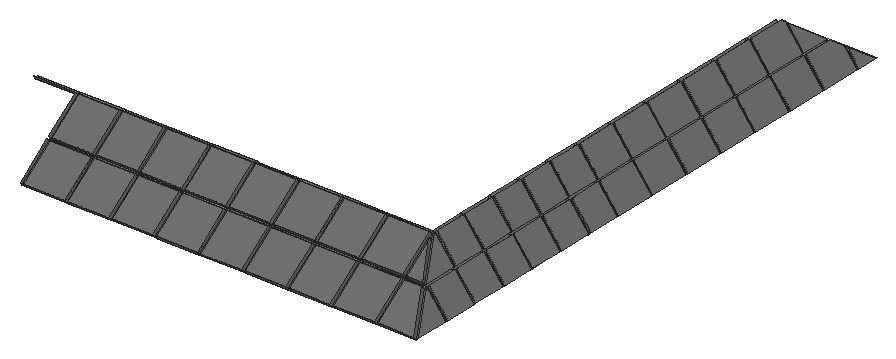
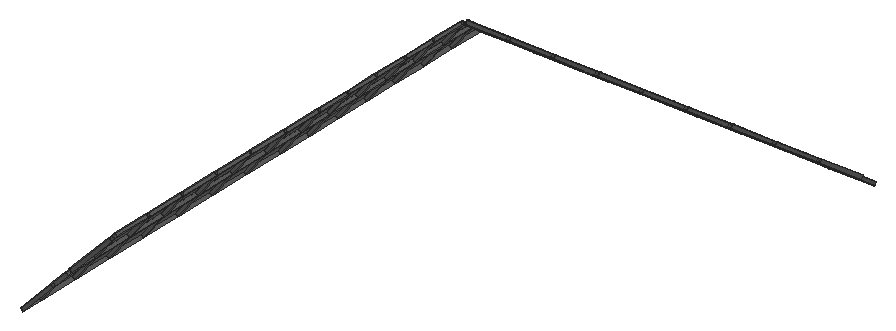
# SketchUp Ruby script. Lengths in inches.
U = 1.inch
M = Sketchup.active_model
def pt(a) = Geom::Point3d.new(a.map { |v| v * U })
def face(e, loops, mat)
  f = e.add_face(loops[0].map { |a| pt(a) })
  loops[1..].each { |l| e.add_face(l.map { |a| pt(a) }).erase! }
  f.material = f.back_material = mat if mat
  f
end
# faces: each face lists its corners as indices into pts; further lists are holes
def faces(e, pts, list, mat = nil) = list.each { |f| face(e, (f[0].is_a?(Array) ? f : [f]).map { |l| l.map { |i| pts[i] } }, mat) }
# xy, xz, yz: faces in a plane at the given z, y or x. An outline is a flat list of corners, or four numbers for a rectangle; further outlines are holes
def ring(l) = l.size == 4 ? [[l[0], l[1]], [l[2], l[1]], [l[2], l[3]], [l[0], l[3]]] : l.each_slice(2).to_a
def flat(e, list, mat, &to3) = list.each { |f| face(e, (f[0].is_a?(Array) ? f : [f]).map { |l| ring(l).map { |u, v| to3.(u, v) } }, mat) }
def xy(e, z, list, mat = nil) = flat(e, list, mat) { |x, y| [x, y, z] }
def xz(e, y, list, mat = nil) = flat(e, list, mat) { |x, z| [x, y, z] }
def yz(e, x, list, mat = nil) = flat(e, list, mat) { |y, z| [x, y, z] }
def lines(e, pts, list) = list.each { |a, b| e.add_line(pt(pts[a]), pt(pts[b])) }
# prism: a flat outline (further loops are holes) pulled along v
def prism(e, loops, v, mat = nil)
  f = face(e, loops, mat); d = Geom::Vector3d.new(v.map { |x| x * U })
  f.pushpull(f.normal.samedirection?(d) ? d.length : -d.length)
end
def box(e, o, s, mat = nil) = prism(e, [[o, [o[0] + s[0], o[1], o[2]], [o[0] + s[0], o[1] + s[1], o[2]], [o[0], o[1] + s[1], o[2]]]], [0, 0, s[2]], mat)
def at(x, y, z, deg = 0) = Geom::Transformation.translation(pt([x, y, z])) * Geom::Transformation.rotation(ORIGIN, Z_AXIS, deg.degrees)
def axes(o, x, y, z) = Geom::Transformation.new([*x, 0, *y, 0, *z, 0, *pt(o).to_a, 1])
def part(name) = M.definitions.add(name)
# library, detail: a bought-in or finely detailed component or shape, given as its bounding box
def library(name, o, s) = part(name).tap { |d| box(d.entities, o, s) }
def detail(e, o, s) = box(e.add_group.entities, o, s)
def put(e, d, t, mat = nil) = e.add_instance(d, t).tap { |i| i.material = mat if mat }
def group(e, t, mat = nil) = e.add_group.tap { |g| g.transformation = t; g.material = mat if mat }.entities
root = M.entities
M.materials.add("[Color M05]").color = [114, 114, 114]
xz(root,317.375,[[781.61,416.3,771.3,429.58,772.875,430.81,783.19,417.52]],"[Color M05]")
xz(root,318.58,[[781.61,416.3,783.19,417.52,772.875,430.81,771.3,429.58]],"[Color M05]")
xz(root,336.74,[[781.61,416.3,771.3,429.58,772.875,430.81,783.19,417.52],[770.61,430.47,760.29,443.75,761.87,444.98,772.1875,431.69]],"[Color M05]")
xz(root,337.95,[[781.61,416.3,783.19,417.52,772.875,430.81,771.3,429.58],[770.61,430.47,772.1875,431.69,761.87,444.98,760.29,443.75]],"[Color M05]")
xz(root,356.11,[[781.61,416.3,771.3,429.58,772.875,430.81,783.19,417.52],[770.61,430.47,760.29,443.75,761.87,444.98,772.1875,431.69]],"[Color M05]")
xz(root,357.32,[[781.61,416.3,783.19,417.52,772.875,430.81,771.3,429.58],[770.61,430.47,772.1875,431.69,761.87,444.98,760.29,443.75]],"[Color M05]")
xz(root,375.48,[[781.61,416.3,771.3,429.58,772.875,430.81,783.19,417.52],[770.61,430.47,760.29,443.75,761.87,444.98,772.1875,431.69]],"[Color M05]")
xz(root,376.69,[[781.61,416.3,783.19,417.52,772.875,430.81,771.3,429.58],[770.61,430.47,772.1875,431.69,761.87,444.98,760.29,443.75]],"[Color M05]")
xz(root,394.85,[[781.61,416.3,771.3,429.58,772.875,430.81,783.19,417.52],[770.61,430.47,760.29,443.75,761.87,444.98,772.1875,431.69]],"[Color M05]")
xz(root,396.0625,[[781.61,416.3,783.19,417.52,772.875,430.81,771.3,429.58],[770.61,430.47,772.1875,431.69,761.87,444.98,760.29,443.75]],"[Color M05]")
xz(root,414.22,[[781.61,416.3,771.3,429.58,772.875,430.81,783.19,417.52],[770.61,430.47,760.29,443.75,761.87,444.98,772.1875,431.69]],"[Color M05]")
xz(root,415.43,[[781.61,416.3,783.19,417.52,772.875,430.81,771.3,429.58],[770.61,430.47,772.1875,431.69,761.87,444.98,760.29,443.75]],"[Color M05]")
xz(root,433.59,[[781.61,416.3,771.3,429.58,772.875,430.81,783.19,417.52],[770.61,430.47,760.29,443.75,761.87,444.98,772.1875,431.69]],"[Color M05]")
xz(root,434.8,[[781.61,416.3,783.19,417.52,772.875,430.81,771.3,429.58],[770.61,430.47,772.1875,431.69,761.87,444.98,760.29,443.75]],"[Color M05]")
xz(root,456.8,[[781.61,416.3,771.3,429.58,772.875,430.81,783.19,417.52],[770.61,430.47,760.29,443.75,761.87,444.98,772.1875,431.69]],"[Color M05]")
xz(root,458.01,[[781.61,416.3,783.19,417.52,772.875,430.81,771.3,429.58],[770.61,430.47,772.1875,431.69,761.87,444.98,760.29,443.75]],"[Color M05]")
xz(root,480.02,[[781.61,416.3,771.3,429.58,772.875,430.81,783.19,417.52],[770.61,430.47,760.29,443.75,761.87,444.98,772.1875,431.69]],"[Color M05]")
xz(root,481.23,[[781.61,416.3,783.19,417.52,772.875,430.81,771.3,429.58],[770.61,430.47,772.1875,431.69,761.87,444.98,760.29,443.75]],"[Color M05]")
xz(root,503.23,[[781.61,416.3,771.3,429.58,772.875,430.81,783.19,417.52],[770.61,430.47,760.29,443.75,761.87,444.98,772.1875,431.69]],"[Color M05]")
xz(root,504.44,[[781.61,416.3,783.19,417.52,772.875,430.81,771.3,429.58],[770.61,430.47,772.1875,431.69,761.87,444.98,760.29,443.75]],"[Color M05]")
xz(root,526.45,[[781.61,416.3,771.3,429.58,772.875,430.81,783.19,417.52],[770.61,430.47,760.29,443.75,761.87,444.98,772.1875,431.69]],"[Color M05]")
xz(root,527.66,[[781.61,416.3,783.19,417.52,772.875,430.81,771.3,429.58],[770.61,430.47,772.1875,431.69,761.87,444.98,760.29,443.75]],"[Color M05]")
xz(root,549.66,[[781.61,416.3,771.3,429.58,772.875,430.81,783.19,417.52],[770.61,430.47,760.29,443.75,761.87,444.98,772.1875,431.69]],"[Color M05]")
xz(root,550.86,[[770.61,430.47,772.1875,431.69,761.87,444.98,760.29,443.75]],"[Color M05]")
xz(root,572.875,[[781.61,416.3,771.3,429.58,772.875,430.81,783.19,417.52],[770.61,430.47,761.02,442.82,762.59,444.05,772.1875,431.69]],"[Color M05]")
xz(root,574.08,[[781.61,416.3,783.19,417.52,772.875,430.81,771.3,429.58],[770.61,430.47,772.1875,431.69,763.28,443.16,761.7,441.93]],"[Color M05]")
xz(root,596.09,[[781.61,416.3,774.21,425.84,775.79,427.0625,783.19,417.52]],"[Color M05]")
xz(root,597.3,[[781.61,416.3,783.19,417.52,776.47,426.18,774.89,424.95]],"[Color M05]")
yz(root,568.12,[[299.21,416.3,317.375,429.58,316.19,431.2,298.03,417.91],[318.58,430.47,336.74,443.75,335.5625,445.37,317.4,432.08]],"[Color M05]")
yz(root,569.62,[[299.21,416.3,298.03,417.91,316.19,431.2,317.375,429.58],[318.58,430.47,317.4,432.08,335.5625,445.37,336.74,443.75]],"[Color M05]")
yz(root,592.12,[[299.21,416.3,317.375,429.58,316.19,431.2,298.03,417.91],[318.58,430.47,336.74,443.75,335.5625,445.37,317.4,432.08]],"[Color M05]")
yz(root,593.62,[[299.21,416.3,298.03,417.91,316.19,431.2,317.375,429.58],[318.58,430.47,317.4,432.08,335.5625,445.37,336.74,443.75]],"[Color M05]")
yz(root,616.14,[[318.58,430.47,336.74,443.75,335.5625,445.37,317.4,432.08]],"[Color M05]")
yz(root,616.15,[[299.21,416.3,317.375,429.58,316.19,431.2,298.03,417.91]],"[Color M05]")
yz(root,617.62,[[299.21,416.3,298.03,417.91,316.19,431.2,317.375,429.58],[318.58,430.47,317.4,432.08,335.5625,445.37,336.74,443.75]],"[Color M05]")
yz(root,640.12,[[299.21,416.3,317.375,429.58,316.19,431.2,298.03,417.91],[318.58,430.47,336.74,443.75,335.5625,445.37,317.4,432.08]],"[Color M05]")
yz(root,641.62,[[299.21,416.3,298.03,417.91,316.19,431.2,317.375,429.58],[318.58,430.47,317.4,432.08,335.5625,445.37,336.74,443.75]],"[Color M05]")
yz(root,664.12,[[299.21,416.3,317.375,429.58,316.19,431.2,298.03,417.91],[318.58,430.47,336.74,443.75,335.5625,445.37,317.4,432.08]],"[Color M05]")
yz(root,665.62,[[299.21,416.3,298.03,417.91,316.19,431.2,317.375,429.58],[318.58,430.47,317.4,432.08,335.5625,445.37,336.74,443.75]],"[Color M05]")
yz(root,688.12,[[299.21,416.3,317.375,429.58,316.19,431.2,298.03,417.91],[318.58,430.47,336.74,443.75,335.5625,445.37,317.4,432.08]],"[Color M05]")
yz(root,689.62,[[299.21,416.3,298.03,417.91,316.19,431.2,317.375,429.58],[318.58,430.47,317.4,432.08,335.5625,445.37,336.74,443.75]],"[Color M05]")
yz(root,712.12,[[299.21,416.3,317.375,429.58,316.19,431.2,298.03,417.91],[318.58,430.47,336.74,443.75,335.5625,445.37,317.4,432.08]],"[Color M05]")
yz(root,713.62,[[299.21,416.3,298.03,417.91,316.19,431.2,317.375,429.58],[318.58,430.47,317.4,432.08,335.5625,445.37,336.74,443.75]],"[Color M05]")
yz(root,736.12,[[299.21,416.3,317.375,429.58,316.19,431.2,298.03,417.91],[318.58,430.47,336.74,443.75,335.5625,445.37,317.4,432.08]],"[Color M05]")
yz(root,737.62,[[299.21,416.3,298.03,417.91,316.19,431.2,317.375,429.58],[318.58,430.47,317.4,432.08,335.5625,445.37,336.74,443.75]],"[Color M05]")
yz(root,760.12,[[299.21,416.3,317.375,429.58,316.19,431.2,298.03,417.91]],"[Color M05]")
yz(root,761.62,[[299.21,416.3,298.03,417.91,316.19,431.2,317.375,429.58],[318.58,430.47,317.4,432.08,333.22,443.65,334.4,442.04]],"[Color M05]")
p = [[569.62,299.21,416.3],[592.12,299.21,416.3],[592.12,298.03,417.91],[569.62,298.03,417.91],[593.62,299.21,416.3],[616.15,299.21,416.3],
  [616.15,298.03,417.91],[593.62,298.03,417.91],[617.62,299.21,416.3],[640.12,299.21,416.3],[640.12,298.03,417.91],[617.62,298.03,417.91],
  [641.62,299.21,416.3],[664.12,299.21,416.3],[664.12,298.03,417.91],[641.62,298.03,417.91],[665.62,299.21,416.3],[688.12,299.21,416.3],
  [688.12,298.03,417.91],[665.62,298.03,417.91],[689.62,299.21,416.3],[712.12,299.21,416.3],[712.12,298.03,417.91],[689.62,298.03,417.91],
  [713.62,299.21,416.3],[736.12,299.21,416.3],[736.12,298.03,417.91],[713.62,298.03,417.91],[737.62,299.21,416.3],[760.12,299.21,416.3],
  [760.12,298.03,417.91],[737.62,298.03,417.91],[761.62,299.21,416.3],[781.61,299.21,416.3],[781.61,298.03,417.91],[761.62,298.03,417.91],
  [771.3,317.375,429.58],[771.3,316.19,431.2],[568.12,299.21,416.3],[569.62,317.375,429.58],[568.12,317.375,429.58],[593.62,317.375,429.58],
  [592.12,317.375,429.58],[617.62,317.375,429.58],[616.15,317.375,429.58],[641.62,317.375,429.58],[640.12,317.375,429.58],[665.62,317.375,429.58],
  [664.12,317.375,429.58],[689.62,317.375,429.58],[688.12,317.375,429.58],[713.62,317.375,429.58],[712.12,317.375,429.58],[737.62,317.375,429.58],
  [736.12,317.375,429.58],[761.62,317.375,429.58],[760.12,317.375,429.58],[783.19,299.21,417.52],[772.875,317.375,430.81],[781.61,317.375,416.3],
  [783.19,317.375,417.52],[781.61,318.58,416.3],[771.3,318.58,429.58],[781.61,336.74,416.3],[783.19,336.74,417.52],[783.19,318.58,417.52],
  [781.61,337.95,416.3],[771.3,337.95,429.58],[771.3,336.74,429.58],[781.61,356.11,416.3],[783.19,356.11,417.52],[783.19,337.95,417.52],
  [781.61,357.32,416.3],[771.3,357.32,429.58],[771.3,356.11,429.58],[781.61,375.48,416.3],[783.19,375.48,417.52],[783.19,357.32,417.52],
  [781.61,376.69,416.3],[771.3,376.69,429.58],[771.3,375.48,429.58],[781.61,394.85,416.3],[783.19,394.85,417.52],[783.19,376.69,417.52],
  [781.61,396.0625,416.3],[771.3,396.0625,429.58],[771.3,394.85,429.58],[781.61,414.22,416.3],[783.19,414.22,417.52],[783.19,396.0625,417.52],
  [781.61,415.43,416.3],[771.3,415.43,429.58],[771.3,414.22,429.58],[781.61,433.59,416.3],[783.19,433.59,417.52],[783.19,415.43,417.52],
  [781.61,434.8,416.3],[771.3,434.8,429.58],[771.3,433.59,429.58],[781.61,456.8,416.3],[783.19,456.8,417.52],[783.19,434.8,417.52],
  [781.61,458.01,416.3],[771.3,458.01,429.58],[771.3,456.8,429.58],[781.61,480.02,416.3],[783.19,480.02,417.52],[783.19,458.01,417.52],
  [781.61,481.23,416.3],[771.3,481.23,429.58],[771.3,480.02,429.58],[781.61,503.23,416.3],[783.19,503.23,417.52],[783.19,481.23,417.52],
  [781.61,504.44,416.3],[771.3,504.44,429.58],[771.3,503.23,429.58],[781.61,526.45,416.3],[783.19,526.45,417.52],[783.19,504.44,417.52],
  [781.61,527.66,416.3],[771.3,527.66,429.58],[771.3,526.45,429.58],[781.61,549.66,416.3],[783.19,549.66,417.52],[783.19,527.66,417.52],
  [781.61,550.87,416.3],[771.3,550.86,429.58],[771.3,549.66,429.58],[783.19,550.87,417.52],[772.875,550.86,430.81],[781.61,572.875,416.3],
  [783.19,572.875,417.52],[781.61,574.08,416.3],[771.3,574.08,429.58],[771.3,572.875,429.58],[781.61,596.09,416.3],[783.19,596.09,417.52],
  [783.19,574.08,417.52],[781.61,597.3,416.3],[774.89,597.3,424.95],[774.21,596.09,425.84],[781.61,609.125,416.3],[776.47,597.3,426.18],
  [783.19,609.125,417.52],[783.19,597.3,417.52],[772.875,336.74,430.81],[772.875,318.58,430.81],[772.875,356.11,430.81],[772.875,337.95,430.81],
  [772.875,375.48,430.81],[772.875,357.32,430.81],[772.875,394.85,430.81],[772.875,376.69,430.81],[772.875,414.22,430.81],[772.875,396.0625,430.81],
  [772.875,433.59,430.81],[772.875,415.43,430.81],[772.875,456.8,430.81],[772.875,434.8,430.81],[772.875,480.02,430.81],[772.875,458.01,430.81],
  [772.875,503.23,430.81],[772.875,481.23,430.81],[772.875,526.45,430.81],[772.875,504.44,430.81],[772.875,549.66,430.81],[772.875,527.66,430.81],
  [772.875,572.875,430.81],[775.79,596.09,427.0625],[772.875,590.97,430.81],[772.875,574.08,430.81],[592.12,316.19,431.2],[569.62,316.19,431.2],
  [616.15,316.19,431.2],[593.62,316.19,431.2],[640.12,316.19,431.2],[617.62,316.19,431.2],[664.12,316.19,431.2],[641.62,316.19,431.2],
  [688.12,316.19,431.2],[665.62,316.19,431.2],[712.12,316.19,431.2],[689.62,316.19,431.2],[736.12,316.19,431.2],[713.62,316.19,431.2],
  [760.12,316.19,431.2],[737.62,316.19,431.2],[761.62,316.19,431.2],[771.3,590.97,429.58],[569.62,318.58,430.47],[568.12,318.58,430.47],
  [592.12,318.58,430.47],[593.62,318.58,430.47],[616.14,318.58,430.47],[617.62,318.58,430.47],[640.12,318.58,430.47],[641.62,318.58,430.47],
  [664.12,318.58,430.47],[665.62,318.58,430.47],[688.12,318.58,430.47],[689.62,318.58,430.47],[712.12,318.58,430.47],[713.62,318.58,430.47],
  [736.12,318.58,430.47],[737.62,318.58,430.47],[760.12,318.58,430.47],[761.62,318.58,430.47],[770.61,318.58,430.47],[770.61,336.74,430.47],
  [770.61,337.95,430.47],[770.61,356.11,430.47],[770.61,357.32,430.47],[770.61,375.48,430.47],[770.61,376.69,430.47],[770.61,394.85,430.47],
  [770.61,396.0625,430.47],[770.61,414.22,430.47],[770.61,415.43,430.47],[770.61,433.59,430.47],[770.61,434.8,430.47],[770.61,456.8,430.47],
  [770.61,458.01,430.47],[770.61,480.02,430.47],[770.61,481.23,430.47],[770.61,503.23,430.47],[770.61,504.44,430.47],[770.61,526.45,430.47],
  [770.61,527.66,430.47],[770.61,549.66,430.47],[770.61,550.86,430.47],[770.61,572.875,430.47],[770.61,574.08,430.47],[770.61,589.76,430.47],
  [592.12,317.4,432.08],[569.62,317.4,432.08],[616.14,317.4,432.08],[593.62,317.4,432.08],[640.12,317.4,432.08],[617.62,317.4,432.08],
  [664.12,317.4,432.08],[641.62,317.4,432.08],[688.12,317.4,432.08],[665.62,317.4,432.08],[712.12,317.4,432.08],[689.62,317.4,432.08],
  [736.12,317.4,432.08],[713.62,317.4,432.08],[760.12,317.4,432.08],[737.62,317.4,432.08],[760.11,336.74,443.75],[760.11,335.5625,445.37],
  [761.62,334.4,442.04],[761.62,333.22,443.65],[770.61,317.4,432.08],[761.62,317.4,432.08],[569.62,336.74,443.75],[568.12,336.74,443.75],
  [593.62,336.74,443.75],[592.12,336.74,443.75],[617.62,336.74,443.75],[616.14,336.74,443.75],[641.62,336.74,443.75],[640.12,336.74,443.75],
  [665.62,336.74,443.75],[664.12,336.74,443.75],[689.62,336.74,443.75],[688.12,336.74,443.75],[713.62,336.74,443.75],[712.12,336.74,443.75],
  [737.62,336.74,443.75],[736.12,336.74,443.75],[760.29,336.74,443.75],[772.1875,318.58,431.69],[763.2,334.4,443.26],[772.1875,336.74,431.69],
  [760.29,337.95,443.75],[772.1875,356.11,431.69],[772.1875,337.95,431.69],[760.29,357.32,443.75],[760.29,356.11,443.75],[772.1875,375.48,431.69],
  [772.1875,357.32,431.69],[760.29,376.69,443.75],[760.29,375.48,443.75],[772.1875,394.85,431.69],[772.1875,376.69,431.69],[760.29,396.0625,443.75],
  [760.29,394.85,443.75],[772.1875,414.22,431.69],[772.1875,396.0625,431.69],[760.29,415.43,443.75],[760.29,414.22,443.75],[772.1875,433.59,431.69],
  [772.1875,415.43,431.69],[760.29,434.8,443.75],[760.29,433.59,443.75],[772.1875,456.8,431.69],[772.1875,434.8,431.69],[760.29,458.01,443.75],
  [760.29,456.8,443.75],[772.1875,480.02,431.69],[772.1875,458.01,431.69],[760.29,481.23,443.75],[760.29,480.02,443.75],[772.1875,503.23,431.69],
  [772.1875,481.23,431.69],[760.29,504.44,443.75],[760.29,503.23,443.75],[772.1875,526.45,431.69],[772.1875,504.44,431.69],[760.29,527.66,443.75],
  [760.29,526.45,443.75],[772.1875,549.66,431.69],[772.1875,527.66,431.69],[760.29,550.86,443.75],[760.29,549.66,443.75],[772.1875,572.875,431.69],
  [772.1875,550.86,431.69],[761.7,574.08,441.93],[761.02,572.875,442.82],[763.28,574.08,443.16],[772.1875,589.76,431.69],[772.1875,574.08,431.69],
  [761.87,336.74,444.98],[761.87,356.11,444.98],[761.87,337.95,444.98],[761.87,375.48,444.98],[761.87,357.32,444.98],[761.87,394.85,444.98],
  [761.87,376.69,444.98],[761.87,414.22,444.98],[761.87,396.0625,444.98],[761.87,433.59,444.98],[761.87,415.43,444.98],[761.87,456.8,444.98],
  [761.87,434.8,444.98],[761.87,480.02,444.98],[761.87,458.01,444.98],[761.87,503.23,444.98],[761.87,481.23,444.98],[761.87,526.45,444.98],
  [761.87,504.44,444.98],[761.87,549.66,444.98],[761.87,527.66,444.98],[762.59,572.875,444.05],[761.87,571.6,444.98],[761.87,550.86,444.98],
  [592.12,335.5625,445.37],[569.62,335.5625,445.37],[616.14,335.5625,445.37],[593.62,335.5625,445.37],[640.12,335.5625,445.37],[617.62,335.5625,445.37],
  [664.12,335.5625,445.37],[641.62,335.5625,445.37],[688.12,335.5625,445.37],[665.62,335.5625,445.37],[712.12,335.5625,445.37],[689.62,335.5625,445.37],
  [736.12,335.5625,445.37],[713.62,335.5625,445.37],[737.62,335.5625,445.37],[760.29,571.6,443.75],[545.62,336.74,443.75],[545.62,335.5625,445.37],
  [568.12,335.5625,445.37],[568.12,337.95,444.64],[545.62,337.95,444.64],[569.62,337.95,444.64],[592.12,337.95,444.64],[593.62,337.95,444.64],
  [616.14,337.95,444.64],[617.62,337.95,444.64],[640.12,337.95,444.64],[641.62,337.95,444.64],[664.12,337.95,444.64],[665.62,337.95,444.64],
  [688.12,337.95,444.64],[689.62,337.95,444.64],[712.12,337.95,444.64],[713.62,337.95,444.64],[736.12,337.95,444.64],[737.62,337.95,444.64],
  [760.11,337.06,443.98],[759.6,337.95,444.64],[759.6,356.11,444.64],[759.6,357.32,444.64],[759.6,375.48,444.64],[759.6,376.69,444.64],
  [759.6,394.85,444.64],[759.6,396.0625,444.64],[759.6,414.22,444.64],[759.6,415.43,444.64],[759.6,433.59,444.64],[759.6,434.8,444.64],
  [759.6,456.8,444.64],[759.6,458.01,444.64],[759.6,480.02,444.64],[759.6,481.23,444.64],[759.6,503.23,444.64],[759.6,504.44,444.64],
  [759.6,526.45,444.64],[759.6,527.66,444.64],[759.6,549.66,444.64],[759.6,550.86,444.64],[759.6,570.39,444.64]]
faces(root,p,[[0,1,2,3],[4,5,6,7],[8,9,10,11],[12,13,14,15],[16,17,18,19],[20,21,22,23],[24,25,26,27],[28,29,30,31],
  [32,33,34,35],[33,36,37,34],[38,0,39,40],[1,4,41,42],[5,8,43,44],[9,12,45,46],[13,16,47,48],[17,20,49,50],
  [21,24,51,52],[25,28,53,54],[29,32,55,56],[36,33,57,58],[33,59,60,57],[61,62,36,59],[61,63,64,65],[63,66,67,68],
  [66,69,70,71],[69,72,73,74],[72,75,76,77],[75,78,79,80],[78,81,82,83],[81,84,85,86],[84,87,88,89],[87,90,91,92],
  [90,93,94,95],[93,96,97,98],[96,99,100,101],[99,102,103,104],[102,105,106,107],[105,108,109,110],[108,111,112,113],[111,114,115,116],
  [114,117,118,119],[117,120,121,122],[120,123,124,125],[123,126,127,128],[127,126,129,130],[126,131,132,129],[131,133,134,135],[133,136,137,138],
  [136,139,140,141],[142,140,143,144],[139,142,144,145],[57,60,58],[65,64,146,147],[71,70,148,149],[77,76,150,151],[83,82,152,153],
  [89,88,154,155],[95,94,156,157],[101,100,158,159],[107,106,160,161],[113,112,162,163],[119,118,164,165],[125,124,166,167],[129,132,168,130],
  [138,137,169,170,171],[144,143,145],[3,2,172,173],[7,6,174,175],[11,10,176,177],[15,14,178,179],[19,18,180,181],[23,22,182,183],
  [27,26,184,185],[31,30,186,187],[37,188,35,34],[141,189,170,169],[42,39,173,172],[44,41,175,174],[46,43,177,176],[48,45,179,178],
  [50,47,181,180],[52,49,183,182],[54,51,185,184],[56,53,187,186],[36,55,188,37],[40,39,190,191],[39,42,192,190],[42,41,193,192],
  [41,44,194,193],[44,43,195,194],[43,46,196,195],[46,45,197,196],[45,48,198,197],[48,47,199,198],[47,50,200,199],[50,49,201,200],
  [49,52,202,201],[52,51,203,202],[51,54,204,203],[54,53,205,204],[53,56,206,205],[56,55,207,206],[208,207,55,36],[208,36,62],
  [62,68,209,208],[68,62,147,146],[68,67,210,209],[67,74,211,210],[74,67,149,148],[74,73,212,211],[73,80,213,212],[80,73,151,150],
  [80,79,214,213],[79,86,215,214],[86,79,153,152],[86,85,216,215],[85,92,217,216],[92,85,155,154],[92,91,218,217],[91,98,219,218],
  [98,91,157,156],[98,97,220,219],[97,104,221,220],[104,97,159,158],[104,103,222,221],[103,110,223,222],[110,103,161,160],[110,109,224,223],
  [109,116,225,224],[116,109,163,162],[116,115,226,225],[115,122,227,226],[122,115,165,164],[122,121,228,227],[121,128,229,228],[128,121,167,166],
  [128,127,230,229],[127,135,231,230],[135,127,130,168],[135,134,232,231],[233,232,134,189],[189,134,171,170],[190,192,234,235],[193,194,236,237],
  [195,196,238,239],[197,198,240,241],[199,200,242,243],[201,202,244,245],[203,204,246,247],[205,206,248,249],[206,250,251,248],[208,252,253,254],
  [207,208,254,255],[191,190,256,257],[192,193,258,259],[194,195,260,261],[196,197,262,263],[198,199,264,265],[200,201,266,267],[202,203,268,269],
  [204,205,270,271],[206,207,252,272,250],[252,208,273,274],[208,209,275,273],[210,276,272,209],[210,211,277,278],[212,279,280,211],[212,213,281,282],
  [214,283,284,213],[214,215,285,286],[215,216,287,288],[216,217,289,290],[217,218,291,292],[218,219,293,294],[219,220,295,296],[220,221,297,298],
  [221,222,299,300],[222,223,301,302],[223,224,303,304],[224,225,305,306],[225,226,307,308],[226,227,309,310],[227,228,311,312],[228,229,313,314],
  [229,230,315,316],[230,231,317,318],[231,232,319,320],[233,319,321,322],[232,233,322,323],[273,275,324,274],[277,325,326,278],[281,327,328,282],
  [286,285,329,330],[290,289,331,332],[294,293,333,334],[298,297,335,336],[302,301,337,338],[306,305,339,340],[310,309,341,342],[314,313,343,344],
  [318,317,345,346,347],[322,321,323],[235,234,348,349],[237,236,350,351],[239,238,352,353],[241,240,354,355],[243,242,356,357],[245,244,358,359],
  [247,246,360,361],[249,248,251,362],[254,253,255],[272,252,274,324],[320,363,346,345],[257,364,365,366],[259,256,349,348],[261,258,351,350],
  [263,260,353,352],[265,262,355,354],[267,264,357,356],[269,266,359,358],[271,268,361,360],[250,270,362,251],[364,257,367,368],[257,256,369,367],
  [256,259,370,369],[259,258,371,370],[258,261,372,371],[261,260,373,372],[260,263,374,373],[263,262,375,374],[262,265,376,375],[265,264,377,376],
  [264,267,378,377],[267,266,379,378],[266,269,380,379],[269,268,381,380],[268,271,382,381],[271,270,383,382],[270,250,384,385,383],[384,272,276,385],
  [272,384,250],[280,386,385,276],[280,276,326,325],[279,387,386,280],[284,388,387,279],[284,279,328,327],[283,389,388,284],[283,288,390,389],
  [288,283,330,329],[288,287,391,390],[287,292,392,391],[292,287,332,331],[292,291,393,392],[291,296,394,393],[296,291,334,333],[296,295,395,394],
  [295,300,396,395],[300,295,336,335],[300,299,397,396],[299,304,398,397],[304,299,338,337],[304,303,399,398],[303,308,400,399],[308,303,340,339],
  [308,307,401,400],[307,312,402,401],[312,307,342,341],[312,311,403,402],[311,316,404,403],[316,311,344,343],[316,315,405,404],[406,405,315,363],
  [363,315,347,346]],"[Color M05]")
